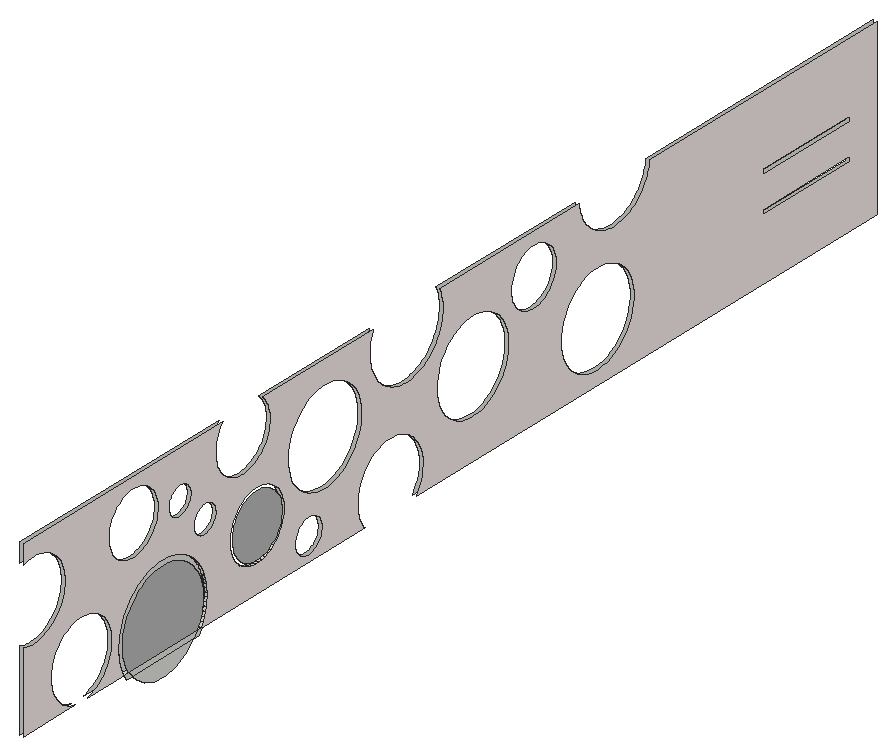
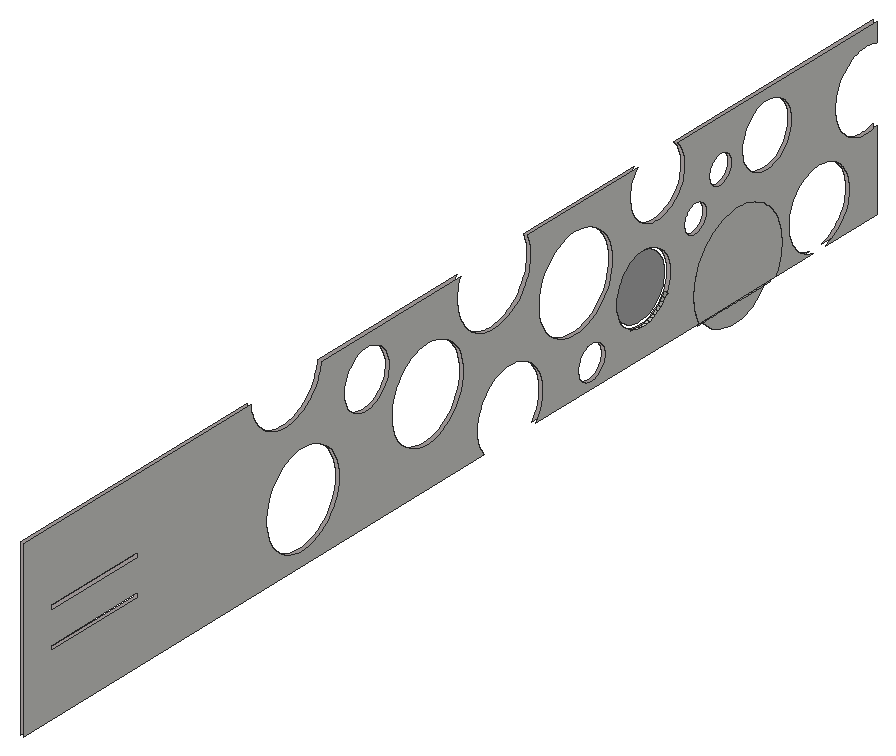
# SketchUp Ruby script. Lengths in inches.
U = 1.inch
M = Sketchup.active_model
def pt(a) = Geom::Point3d.new(a.map { |v| v * U })
def face(e, loops, mat)
  f = e.add_face(loops[0].map { |a| pt(a) })
  loops[1..].each { |l| e.add_face(l.map { |a| pt(a) }).erase! }
  f.material = f.back_material = mat if mat
  f
end
# faces: each face lists its corners as indices into pts; further lists are holes
def faces(e, pts, list, mat = nil) = list.each { |f| face(e, (f[0].is_a?(Array) ? f : [f]).map { |l| l.map { |i| pts[i] } }, mat) }
# xy, xz, yz: faces in a plane at the given z, y or x. An outline is a flat list of corners, or four numbers for a rectangle; further outlines are holes
def ring(l) = l.size == 4 ? [[l[0], l[1]], [l[2], l[1]], [l[2], l[3]], [l[0], l[3]]] : l.each_slice(2).to_a
def flat(e, list, mat, &to3) = list.each { |f| face(e, (f[0].is_a?(Array) ? f : [f]).map { |l| ring(l).map { |u, v| to3.(u, v) } }, mat) }
def xy(e, z, list, mat = nil) = flat(e, list, mat) { |x, y| [x, y, z] }
def xz(e, y, list, mat = nil) = flat(e, list, mat) { |x, z| [x, y, z] }
def yz(e, x, list, mat = nil) = flat(e, list, mat) { |y, z| [x, y, z] }
def lines(e, pts, list) = list.each { |a, b| e.add_line(pt(pts[a]), pt(pts[b])) }
# prism: a flat outline (further loops are holes) pulled along v
def prism(e, loops, v, mat = nil)
  f = face(e, loops, mat); d = Geom::Vector3d.new(v.map { |x| x * U })
  f.pushpull(f.normal.samedirection?(d) ? d.length : -d.length)
end
def box(e, o, s, mat = nil) = prism(e, [[o, [o[0] + s[0], o[1], o[2]], [o[0] + s[0], o[1] + s[1], o[2]], [o[0], o[1] + s[1], o[2]]]], [0, 0, s[2]], mat)
def at(x, y, z, deg = 0) = Geom::Transformation.translation(pt([x, y, z])) * Geom::Transformation.rotation(ORIGIN, Z_AXIS, deg.degrees)
def axes(o, x, y, z) = Geom::Transformation.new([*x, 0, *y, 0, *z, 0, *pt(o).to_a, 1])
def part(name) = M.definitions.add(name)
# library, detail: a bought-in or finely detailed component or shape, given as its bounding box
def library(name, o, s) = part(name).tap { |d| box(d.entities, o, s) }
def detail(e, o, s) = box(e.add_group.entities, o, s)
def put(e, d, t, mat = nil) = e.add_instance(d, t).tap { |i| i.material = mat if mat }
def group(e, t, mat = nil) = e.add_group.tap { |g| g.transformation = t; g.material = mat if mat }.entities
root = M.entities
M.materials.add("Generic\#2").color = [246, 234, 234]
M.materials.add("[Mirror 01]").color = [185, 185, 185]
xy(root,46.5,[[9,53.23,10.6875,94.93]])
yz(root,9,[[[0.4375,46.5,0.4375,80.35,1.09,80.07,2.53,79.73,3.92,79.53,5.3125,79.45,6.71,79.48,8.1,79.625,9.48,79.89,10.83,80.27,12.14,80.75,13.4,81.35,14.61,82.05,15.76,82.85,16.84,83.74,17.84,84.72,18.75,85.78,19.58,86.91,20.3,88.11,20.92,89.36,21.44,90.66,21.84,92,22.14,93.37,22.3125,94.76,22.375,96.15,22.32,97.55,22.14,98.94,21.85,100.31,21.45,101.65,20.9375,102.95,20.32,104.21,19.6,105.4,18.78,106.54,17.86,107.6,16.87,108.58,15.79,109.47,14.64,110.28,13.43,110.98,12.17,111.58,10.86,112.07,9.51,112.45,8.14,112.71,6.75,112.87,5.35,112.9,3.95,112.82,2.57,112.62,1.18,112.3,0.4375,112.04,0.4375,120,106.01,120,105.5,119.44,104.63,118.3125,103.89,117.11,103.26,115.84,102.75,114.51,102.38,113.14,102.14,111.74,102.04,110.32,102.07,108.91,102.24,107.5,102.55,106.11,102.99,104.76,103.56,103.46,104.25,102.22,105.05,101.05,105.97,99.97,106.98,98.97,108.09,98.09,109.28,97.31,110.53,96.65,111.85,96.11,113.21,95.71,114.6,95.43,116.01,95.3,117.43,95.3,118.85,95.43,120.24,95.71,121.6,96.11,122.91,96.65,124.17,97.31,125.36,98.09,126.46,98.97,127.48,99.97,128.4,101.05,129.2,102.22,129.89,103.46,130.46,104.76,130.9,106.11,131.2,107.5,131.375,108.91,131.41,110.32,131.31,111.74,131.07,113.14,130.69,114.51,130.19,115.84,129.5625,117.11,128.8125,118.3125,127.95,119.44,127.43,120,185.75,120,185.61,119.71,185.04,118.26,184.59,116.77,184.25,115.24,184.04,113.7,183.95,112.14,183.99,110.58,184.15,109.02,184.43,107.49,184.84,105.98,185.36,104.51,185.99,103.08,186.74,101.71,187.6,100.41,188.55,99.17,189.6,98.02,190.74,96.95,191.96,95.97,193.25,95.1,194.61,94.33,196.02,93.67,197.48,93.12,198.99,92.69,200.52,92.38,202.07,92.2,203.625,92.14,205.19,92.2,206.74,92.38,208.27,92.69,209.77,93.12,211.23,93.67,212.64,94.33,214,95.1,215.29,95.97,216.51,96.95,217.65,98.02,218.7,99.17,219.66,100.41,220.51,101.71,221.26,103.08,221.89,104.51,222.42,105.98,222.82,107.49,223.1,109.02,223.26,110.58,223.3,112.14,223.21,113.7,223,115.24,222.66,116.77,222.21,118.26,221.64,119.71,221.5,120,295.22,120,295.4375,118.67,295.65,117.68,295.91,116.7,296.23,115.73,296.6,114.78,297.02,113.85,297.49,112.95,298,112.07,298.56,111.23,299.17,110.41,299.82,109.625,300.51,108.875,301.24,108.17,302,107.5,302.8,106.87,303.63,106.28,304.49,105.74,305.38,105.25,306.3,104.8,307.24,104.41,308.19,104.06,309.17,103.77,310.15,103.52,311.15,103.34,312.16,103.2,313.18,103.12,314.19,103.09,315.21,103.12,316.22,103.2,317.23,103.34,318.23,103.52,319.22,103.77,320.19,104.06,321.15,104.41,322.09,104.8,323,105.25,323.89,105.74,324.75,106.28,325.59,106.87,326.39,107.5,327.15,108.17,327.88,108.875,328.57,109.625,329.22,110.41,329.82,111.23,330.38,112.07,330.9,112.95,331.37,113.85,331.79,114.78,332.15,115.73,332.47,116.7,332.74,117.68,332.95,118.67,333.16,120,453.375,120,453.375,46.5,209.04,46.5,209.84,47.59,210.84,49.33,211.63,51.17,212.21,53.09,212.56,55.07,212.6875,57.07,212.58,59.07,212.25,61.05,211.7,62.97,210.93,64.82,209.95,66.58,208.78,68.2,207.4375,69.69,205.93,71.01,204.28,72.15,202.51,73.1,200.65,73.84,198.71,74.36,196.73,74.65,194.73,74.72,192.73,74.5625,190.76,74.18,188.85,73.57,187.02,72.74,185.3,71.72,183.7,70.5,182.26,69.11,180.98,67.57,179.89,65.89,178.99,64.1,178.31,62.21,177.84,60.26,177.6,58.27,177.59,56.27,177.81,54.27,178.25,52.32,178.91,50.42,179.79,48.62,180.86,46.93,181.21,46.5,94.93,46.5,94.96,46.54,95.8,48.26,96.46,49.91,96.99,51.61,97.4,53.35,97.67,55.1,97.8125,56.88,97.82,58.66,97.7,60.4375,97.44,62.2,97.05,63.93,96.53,65.64,95.89,67.3,95.125,68.91,94.24,70.45,93.24,71.92,92.14,73.32,90.93,74.63,89.63,75.84,88.24,76.96,86.77,77.97,85.23,78.86,83.63,79.64,81.97,80.29,80.27,80.82,78.54,81.22,76.78,81.49,75,81.625,73.22,81.63,71.45,81.5,69.69,81.23,67.95,80.84,66.25,80.32,64.59,79.67,62.98,78.9,61.44,78.01,59.97,77,58.58,75.89,57.27,74.68,56.0625,73.38,54.95,71.99,53.95,70.52,53.06,68.97,52.29,67.37,51.64,65.71,51.12,64.01,50.72,62.27,50.46,60.51,50.33,58.74,50.33,56.96,50.47,55.18,50.73,53.42,51.13,51.69,51.66,49.99,52.32,48.33,53.12,46.68,53.23,46.5,34.125,46.5,35.01,46.69,36.33,47.11,37.61,47.625,38.84,48.25,40.02,48.99,41.125,49.8125,42.16,50.73,43.11,51.73,43.98,52.8125,44.75,53.96,45.42,55.17,45.98,56.4375,46.43,57.74,46.78,59.08,47,60.45,47.12,61.83,47.11,63.21,46.99,64.59,46.75,65.95,46.39,67.29,45.93,68.59,45.35,69.85,44.67,71.05,43.89,72.19,43.02,73.27,42.06,74.26,41.01,75.17,39.9,75.99,38.72,76.71,37.48,77.32,36.19,77.83,34.87,78.23,33.51,78.52,32.14,78.6875,30.76,78.74,29.38,78.68,28.01,78.49,26.66,78.2,25.34,77.79,24.05,77.26,22.82,76.64,21.65,75.91,20.54,75.08,19.5,74.16,18.55,73.16,17.6875,72.08,16.92,70.93,16.25,69.72,15.68,68.45,15.23,67.15,14.89,65.81,14.66,64.44,14.55,63.06,14.55,61.68,14.68,60.3,14.92,58.94,15.27,57.6,15.74,56.3,16.3125,55.04,16.99,53.84,17.77,52.7,18.65,51.625,19.61,50.63,20.65,49.72,21.77,48.9,22.95,48.18,24.1875,47.57,25.47,47.06,26.8,46.66,27.54,46.5],[160.49,70.77,162.75,70.92,164.98,71.34,167.15,72,169.22,72.9,171.18,74.04,173,75.39,174.65,76.95,176.12,78.68,177.38,80.56,178.41,82.58,179.21,84.7,179.76,86.9,180.06,89.14,180.1,91.41,179.88,93.66,179.4,95.88,178.68,98.03,177.71,100.08,176.52,102.01,175.12,103.78,173.52,105.39,171.75,106.81,169.83,108.01,167.78,108.99,165.64,109.72,163.43,110.21,161.17,110.44,158.91,110.42,156.66,110.14,154.46,109.6,152.33,108.8125,150.31,107.79,148.42,106.54,146.68,105.09,145.12,103.44,143.75,101.63,142.61,99.68,141.6875,97.61,141.01,95.44,140.59,93.22,140.42,90.96,140.51,88.69,140.86,86.45,141.46,84.27,142.3,82.17,143.38,80.17,144.68,78.32,146.1875,76.62,147.875,75.11,149.72,73.8,151.71,72.71,153.81,71.85,155.99,71.23,158.23,70.87],[305.99,52.23,308.22,52.44,310.42,52.9,312.54,53.61,314.58,54.5625,316.49,55.74,318.25,57.12,319.85,58.7,321.26,60.44,322.45,62.34,323.43,64.36,324.17,66.48,324.66,68.67,324.89,70.9,324.875,73.14,324.6,75.37,324.08,77.55,323.31,79.66,322.3,81.66,321.07,83.54,319.64,85.27,318.02,86.82,316.23,88.17,314.3,89.31,312.25,90.23,310.11,90.91,307.91,91.33,305.68,91.51,303.43,91.43,301.22,91.09,299.05,90.5,296.97,89.67,294.99,88.61,293.15,87.33,291.47,85.85,289.96,84.18,288.66,82.36,287.57,80.39,286.71,78.32,286.1,76.16,285.73,73.95,285.625,71.71,285.77,69.47,286.17,67.26,286.82,65.12,287.71,63.06,288.83,61.11,290.16,59.31,291.69,57.67,293.4,56.21,295.26,54.96,297.25,53.93,299.35,53.13,301.52,52.58,303.74,52.28],[239.61,63.57,241.81,63.77,243.97,64.23,246.06,64.93,248.0625,65.86,249.94,67.02,251.68,68.38,253.25,69.93,254.64,71.65,255.82,73.52,256.77,75.51,257.5,77.59,257.98,79.75,258.22,81.94,258.2,84.15,257.93,86.34,257.41,88.49,256.66,90.5625,255.67,92.54,254.46,94.39,253.05,96.08,251.45,97.61,249.69,98.95,247.79,100.07,245.78,100.97,243.67,101.64,241.5,102.06,239.3,102.23,237.09,102.15,234.91,101.82,232.78,101.24,230.73,100.42,228.78,99.38,226.97,98.12,225.3125,96.66,223.83,95.02,222.55,93.22,221.48,91.29,220.64,89.25,220.03,87.125,219.67,84.95,219.5625,82.74,219.71,80.54,220.1,78.37,220.74,76.25,221.61,74.22,222.71,72.3125,224.03,70.53,225.53,68.92,227.21,67.49,229.05,66.25,231.01,65.24,233.07,64.45,235.21,63.91,237.4,63.61],[123.83,58.04,125.5,58.09,127.15,58.33,128.76,58.76,130.32,59.36,131.8,60.15,133.17,61.09,134.4375,62.1875,135.5625,63.42,136.54,64.77,137.36,66.23,138.01,67.77,138.48,69.375,138.76,71.02,138.85,72.69,138.75,74.36,138.47,76,137.99,77.61,137.34,79.14,136.52,80.6,135.53,81.95,134.4,83.18,133.14,84.27,131.75,85.21,130.28,85.99,128.72,86.59,127.1,87.01,125.45,87.25,123.78,87.29,122.11,87.15,120.48,86.8125,118.89,86.29,117.37,85.6,115.94,84.73,114.62,83.71,113.42,82.54,112.37,81.25,111.47,79.84,110.73,78.34,110.17,76.76,109.8,75.14,109.61,73.48,109.61,71.81,109.8,70.15,110.1875,68.52,110.75,66.95,111.49,65.45,112.4,64.04,113.46,62.75,114.66,61.59,115.98,60.57,117.41,59.71,118.93,59.02,120.52,58.51,122.16,58.18],[59.06,89.02,60.53,89.17,61.96,89.47,63.36,89.93,64.7,90.54,65.96,91.29,67.13,92.18,68.2,93.1875,69.15,94.31,69.97,95.53,70.65,96.83,71.18,98.2,71.5625,99.62,71.78,101.07,71.84,102.54,71.74,104,71.48,105.45,71.06,106.86,70.49,108.21,69.77,109.49,68.92,110.6875,67.93,111.78,66.84,112.76,65.64,113.62,64.36,114.33,63.01,114.9,61.6,115.32,60.15,115.58,58.6875,115.68,57.22,115.62,55.77,115.4,54.35,115.02,52.98,114.48,51.68,113.8,50.46,112.98,49.34,112.03,48.33,110.96,47.44,109.79,46.69,108.53,46.08,107.19,45.625,105.8,45.32,104.36,45.18,102.89,45.2,101.43,45.39,99.97,45.73,98.54,46.22,97.16,46.87,95.84,47.66,94.6,48.58,93.45,49.62,92.41,50.76,91.49,52,90.71,53.32,90.0625,54.71,89.57,56.14,89.23,57.6,89.04],[271.5625,90.52,272.95,90.625,274.32,90.89,275.64,91.3,276.91,91.86,278.11,92.57,279.22,93.41,280.23,94.37,281.125,95.43,281.89,96.59,282.52,97.84,283,99.14,283.33,100.49,283.5,101.87,283.52,103.26,283.37,104.65,283.07,106,282.62,107.32,282.02,108.57,281.28,109.75,280.41,110.84,279.42,111.82,278.33,112.68,277.15,113.41,275.89,114,274.57,114.45,273.21,114.74,271.83,114.87,270.4375,114.85,269.06,114.66,267.71,114.32,266.41,113.83,265.17,113.2,264.01,112.43,262.95,111.53,262,110.51,261.17,109.4,260.47,108.19,259.92,106.92,259.51,105.59,259.26,104.22,259.17,102.83,259.23,101.44,259.45,100.07,259.83,98.73,260.36,97.44,261.03,96.23,261.83,95.09,262.76,94.06,263.8,93.13,264.94,92.34,266.17,91.67,267.46,91.16,268.8,90.79,270.17,90.58],[152.02,49.25,152.83,49.33,153.61,49.5,154.38,49.76,155.11,50.09,155.8,50.51,156.44,51,157.02,51.55,157.54,52.17,157.99,52.84,158.36,53.56,158.65,54.31,158.85,55.09,158.97,55.88,159,56.6875,158.94,57.49,158.79,58.28,158.56,59.06,158.24,59.8,157.85,60.5,157.375,61.15,156.84,61.75,156.23,62.28,155.58,62.75,154.87,63.14,154.13,63.45,153.35,63.67,152.5625,63.81,151.76,63.87,150.95,63.83,150.16,63.7,149.38,63.49,148.63,63.2,147.92,62.82,147.25,62.37,146.64,61.84,146.09,61.26,145.61,60.61,145.2,59.92,144.87,59.18,144.62,58.42,144.46,57.625,144.38,56.82,144.4,56.02,144.5,55.22,144.69,54.4375,144.97,53.68,145.32,52.96,145.76,52.28,146.26,51.65,146.84,51.09,147.47,50.59,148.15,50.16,148.875,49.81,149.63,49.54,150.42,49.36,151.22,49.26],[83.09,93.93,83.68,93.94,84.26,94.02,84.84,94.15,85.4,94.33,85.9375,94.57,86.45,94.86,86.93,95.2,87.38,95.58,87.79,96.01,88.16,96.47,88.48,96.97,88.75,97.49,88.97,98.04,89.14,98.6,89.25,99.18,89.3,99.77,89.3,100.36,89.24,100.95,89.12,101.53,88.95,102.09,88.72,102.64,88.44,103.16,88.12,103.65,87.75,104.11,87.33,104.53,86.88,104.9,86.39,105.24,85.875,105.52,85.33,105.75,84.77,105.93,84.19,106.06,83.61,106.125,83.02,106.13,82.43,106.09,81.85,105.99,81.28,105.83,80.73,105.62,80.2,105.35,79.7,105.04,79.24,104.68,78.81,104.27,78.42,103.83,78.07,103.35,77.78,102.84,77.53,102.3,77.34,101.74,77.2,101.17,77.12,100.59,77.09,100,77.125,99.41,77.21,98.82,77.36,98.25,77.56,97.7,77.81,97.16,78.11,96.66,78.46,96.18,78.85,95.74,79.29,95.34,79.76,94.99,80.26,94.68,80.79,94.42,81.34,94.21,81.91,94.0625,82.5,93.97],[96.4375,81.13,97.02,81.15,97.6,81.23,98.17,81.35,98.72,81.54,99.26,81.77,99.76,82.06,100.24,82.39,100.68,82.77,101.09,83.19,101.45,83.65,101.77,84.14,102.04,84.66,102.25,85.2,102.42,85.76,102.53,86.33,102.58,86.91,102.58,87.49,102.52,88.07,102.4,88.64,102.23,89.2,102.01,89.74,101.73,90.26,101.41,90.74,101.04,91.19,100.64,91.61,100.1875,91.98,99.71,92.3125,99.19,92.59,98.66,92.82,98.1,93,97.53,93.12,96.95,93.1875,96.37,93.2,95.79,93.15,95.22,93.05,94.65,92.9,94.11,92.6875,93.59,92.42,93.1,92.11,92.63,91.76,92.21,91.36,91.83,90.92,91.49,90.45,91.19,89.94,90.95,89.41,90.76,88.86,90.625,88.29,90.54,87.72,90.52,87.13,90.55,86.55,90.64,85.98,90.78,85.41,90.98,84.86,91.22,84.33,91.52,83.83,91.87,83.36,92.26,82.93,92.6875,82.53,93.15,82.18,93.65,81.88,94.17,81.62,94.72,81.42,95.28,81.27,95.86,81.17],[393.02,72.8125,439.14,75],[393.02,88.25,439.14,90.4375]],[53.23,46.5,94.93,46.5,94.96,46.54,95.8,48.26,96.46,49.91,96.99,51.61,97.4,53.35,97.67,55.1,97.8125,56.88,97.82,58.66,97.7,60.4375,97.44,62.2,97.05,63.93,96.53,65.64,95.89,67.3,95.125,68.91,94.24,70.45,93.24,71.92,92.14,73.32,90.93,74.63,89.63,75.84,88.24,76.96,86.77,77.97,85.23,78.86,83.63,79.64,81.97,80.29,80.27,80.82,78.54,81.22,76.78,81.49,75,81.625,73.22,81.63,71.45,81.5,69.69,81.23,67.95,80.84,66.25,80.32,64.59,79.67,62.98,78.9,61.44,78.01,59.97,77,58.58,75.89,57.27,74.68,56.0625,73.38,54.95,71.99,53.95,70.52,53.06,68.97,52.29,67.37,51.64,65.71,51.12,64.01,50.72,62.27,50.46,60.51,50.33,58.74,50.33,56.96,50.47,55.18,50.73,53.42,51.13,51.69,51.66,49.99,52.32,48.33,53.12,46.68]])
yz(root,10.6875,[[75.53,36.56,81,37.66,86,40.14,90.18,43.83,90.37,44.12,57.96,44.12,60.03,41.77,64.67,38.68,69.96,36.9],[54.76,44.12,57.96,44.12,56.33,45.96,56.0625,46.5,53.23,46.5],[57.96,44.12,90.37,44.12,91.96,46.5,56.0625,46.5,56.33,45.96],[90.37,44.12,93.15,44.12,94.93,46.5,91.96,46.5]])
yz(root,10.6875,[[[0.4375,46.5,27.54,46.5,26.8,46.66,25.47,47.06,24.1875,47.57,22.95,48.18,21.77,48.9,20.65,49.72,19.61,50.63,18.65,51.625,17.77,52.7,16.99,53.84,16.3125,55.04,15.74,56.3,15.27,57.6,14.92,58.94,14.68,60.3,14.55,61.68,14.55,63.06,14.66,64.44,14.89,65.81,15.23,67.15,15.68,68.45,16.25,69.72,16.92,70.93,17.6875,72.08,18.55,73.16,19.5,74.16,20.54,75.08,21.65,75.91,22.82,76.64,24.05,77.26,25.34,77.79,26.66,78.2,28.01,78.49,29.38,78.68,30.76,78.74,32.14,78.6875,33.51,78.52,34.87,78.23,36.19,77.83,37.48,77.32,38.72,76.71,39.9,75.99,41.01,75.17,42.06,74.26,43.02,73.27,43.89,72.19,44.67,71.05,45.35,69.85,45.93,68.59,46.39,67.29,46.75,65.95,46.99,64.59,47.11,63.21,47.12,61.83,47,60.45,46.78,59.08,46.43,57.74,45.98,56.4375,45.42,55.17,44.75,53.96,43.98,52.8125,43.11,51.73,42.16,50.73,41.125,49.8125,40.02,48.99,38.84,48.25,37.61,47.625,36.33,47.11,35.01,46.69,34.125,46.5,53.23,46.5,53.12,46.68,52.32,48.33,51.66,49.99,51.13,51.69,50.73,53.42,50.47,55.18,50.33,56.96,50.33,58.74,50.46,60.51,50.72,62.27,51.12,64.01,51.64,65.71,52.29,67.37,53.06,68.97,53.95,70.52,54.95,71.99,56.0625,73.38,57.27,74.68,58.58,75.89,59.97,77,61.44,78.01,62.98,78.9,64.59,79.67,66.25,80.32,67.95,80.84,69.69,81.23,71.45,81.5,73.22,81.63,75,81.625,76.78,81.49,78.54,81.22,80.27,80.82,81.97,80.29,83.63,79.64,85.23,78.86,86.77,77.97,88.24,76.96,89.63,75.84,90.93,74.63,92.14,73.32,93.24,71.92,94.24,70.45,95.125,68.91,95.89,67.3,96.53,65.64,97.05,63.93,97.44,62.2,97.7,60.4375,97.82,58.66,97.8125,56.88,97.67,55.1,97.4,53.35,96.99,51.61,96.46,49.91,95.8,48.26,94.96,46.54,94.93,46.5,181.21,46.5,180.86,46.93,179.79,48.62,178.91,50.42,178.25,52.32,177.81,54.27,177.59,56.27,177.6,58.27,177.84,60.26,178.31,62.21,178.99,64.1,179.89,65.89,180.98,67.57,182.26,69.11,183.7,70.5,185.3,71.72,187.02,72.74,188.85,73.57,190.76,74.18,192.73,74.5625,194.73,74.72,196.73,74.65,198.71,74.36,200.65,73.84,202.51,73.1,204.28,72.15,205.93,71.01,207.4375,69.69,208.78,68.2,209.95,66.58,210.93,64.82,211.7,62.97,212.25,61.05,212.58,59.07,212.6875,57.07,212.56,55.07,212.21,53.09,211.63,51.17,210.84,49.33,209.84,47.59,209.04,46.5,453.375,46.5,453.375,120,333.16,120,332.95,118.67,332.74,117.68,332.47,116.7,332.15,115.73,331.79,114.78,331.37,113.85,330.9,112.95,330.38,112.07,329.82,111.23,329.22,110.41,328.57,109.625,327.88,108.875,327.15,108.17,326.39,107.5,325.59,106.87,324.75,106.28,323.89,105.74,323,105.25,322.09,104.8,321.15,104.41,320.19,104.06,319.22,103.77,318.23,103.52,317.23,103.34,316.22,103.2,315.21,103.12,314.19,103.09,313.18,103.12,312.16,103.2,311.15,103.34,310.15,103.52,309.17,103.77,308.19,104.06,307.24,104.41,306.3,104.8,305.38,105.25,304.49,105.74,303.63,106.28,302.8,106.87,302,107.5,301.24,108.17,300.51,108.875,299.82,109.625,299.17,110.41,298.56,111.23,298,112.07,297.49,112.95,297.02,113.85,296.6,114.78,296.23,115.73,295.91,116.7,295.65,117.68,295.4375,118.67,295.22,120,221.5,120,221.64,119.71,222.21,118.26,222.66,116.77,223,115.24,223.21,113.7,223.3,112.14,223.26,110.58,223.1,109.02,222.82,107.49,222.42,105.98,221.89,104.51,221.26,103.08,220.51,101.71,219.66,100.41,218.7,99.17,217.65,98.02,216.51,96.95,215.29,95.97,214,95.1,212.64,94.33,211.23,93.67,209.77,93.12,208.27,92.69,206.74,92.38,205.19,92.2,203.625,92.14,202.07,92.2,200.52,92.38,198.99,92.69,197.48,93.12,196.02,93.67,194.61,94.33,193.25,95.1,191.96,95.97,190.74,96.95,189.6,98.02,188.55,99.17,187.6,100.41,186.74,101.71,185.99,103.08,185.36,104.51,184.84,105.98,184.43,107.49,184.15,109.02,183.99,110.58,183.95,112.14,184.04,113.7,184.25,115.24,184.59,116.77,185.04,118.26,185.61,119.71,185.75,120,127.43,120,127.95,119.44,128.8125,118.3125,129.5625,117.11,130.19,115.84,130.69,114.51,131.07,113.14,131.31,111.74,131.41,110.32,131.375,108.91,131.2,107.5,130.9,106.11,130.46,104.76,129.89,103.46,129.2,102.22,128.4,101.05,127.48,99.97,126.46,98.97,125.36,98.09,124.17,97.31,122.91,96.65,121.6,96.11,120.24,95.71,118.85,95.43,117.43,95.3,116.01,95.3,114.6,95.43,113.21,95.71,111.85,96.11,110.53,96.65,109.28,97.31,108.09,98.09,106.98,98.97,105.97,99.97,105.05,101.05,104.25,102.22,103.56,103.46,102.99,104.76,102.55,106.11,102.24,107.5,102.07,108.91,102.04,110.32,102.14,111.74,102.38,113.14,102.75,114.51,103.26,115.84,103.89,117.11,104.63,118.3125,105.5,119.44,106.01,120,0.4375,120,0.4375,112.04,1.18,112.3,2.57,112.62,3.95,112.82,5.35,112.9,6.75,112.87,8.14,112.71,9.51,112.45,10.86,112.07,12.17,111.58,13.43,110.98,14.64,110.28,15.79,109.47,16.87,108.58,17.86,107.6,18.78,106.54,19.6,105.4,20.32,104.21,20.9375,102.95,21.45,101.65,21.85,100.31,22.14,98.94,22.32,97.55,22.375,96.15,22.3125,94.76,22.14,93.37,21.84,92,21.44,90.66,20.92,89.36,20.3,88.11,19.58,86.91,18.75,85.78,17.84,84.72,16.84,83.74,15.76,82.85,14.61,82.05,13.4,81.35,12.14,80.75,10.83,80.27,9.48,79.89,8.1,79.625,6.71,79.48,5.3125,79.45,3.92,79.53,2.53,79.73,1.09,80.07,0.4375,80.35],[160.49,70.77,158.23,70.87,155.99,71.23,153.81,71.85,151.71,72.71,149.72,73.8,147.875,75.11,146.1875,76.62,144.68,78.32,143.38,80.17,142.3,82.17,141.46,84.27,140.86,86.45,140.51,88.69,140.42,90.96,140.59,93.22,141.01,95.44,141.6875,97.61,142.61,99.68,143.75,101.63,145.12,103.44,146.68,105.09,148.42,106.54,150.31,107.79,152.33,108.8125,154.46,109.6,156.66,110.14,158.91,110.42,161.17,110.44,163.43,110.21,165.64,109.72,167.78,108.99,169.83,108.01,171.75,106.81,173.52,105.39,175.12,103.78,176.52,102.01,177.71,100.08,178.68,98.03,179.4,95.88,179.88,93.66,180.1,91.41,180.06,89.14,179.76,86.9,179.21,84.7,178.41,82.58,177.38,80.56,176.12,78.68,174.65,76.95,173,75.39,171.18,74.04,169.22,72.9,167.15,72,164.98,71.34,162.75,70.92],[305.99,52.23,303.74,52.28,301.52,52.58,299.35,53.13,297.25,53.93,295.26,54.96,293.4,56.21,291.69,57.67,290.16,59.31,288.83,61.11,287.71,63.06,286.82,65.12,286.17,67.26,285.77,69.47,285.625,71.71,285.73,73.95,286.1,76.16,286.71,78.32,287.57,80.39,288.66,82.36,289.96,84.18,291.47,85.85,293.15,87.33,294.99,88.61,296.97,89.67,299.05,90.5,301.22,91.09,303.43,91.43,305.68,91.51,307.91,91.33,310.11,90.91,312.25,90.23,314.3,89.31,316.23,88.17,318.02,86.82,319.64,85.27,321.07,83.54,322.3,81.66,323.31,79.66,324.08,77.55,324.6,75.37,324.875,73.14,324.89,70.9,324.66,68.67,324.17,66.48,323.43,64.36,322.45,62.34,321.26,60.44,319.85,58.7,318.25,57.12,316.49,55.74,314.58,54.5625,312.54,53.61,310.42,52.9,308.22,52.44],[239.61,63.57,237.4,63.61,235.21,63.91,233.07,64.45,231.01,65.24,229.05,66.25,227.21,67.49,225.53,68.92,224.03,70.53,222.71,72.3125,221.61,74.22,220.74,76.25,220.1,78.37,219.71,80.54,219.5625,82.74,219.67,84.95,220.03,87.125,220.64,89.25,221.48,91.29,222.55,93.22,223.83,95.02,225.3125,96.66,226.97,98.12,228.78,99.38,230.73,100.42,232.78,101.24,234.91,101.82,237.09,102.15,239.3,102.23,241.5,102.06,243.67,101.64,245.78,100.97,247.79,100.07,249.69,98.95,251.45,97.61,253.05,96.08,254.46,94.39,255.67,92.54,256.66,90.5625,257.41,88.49,257.93,86.34,258.2,84.15,258.22,81.94,257.98,79.75,257.5,77.59,256.77,75.51,255.82,73.52,254.64,71.65,253.25,69.93,251.68,68.38,249.94,67.02,248.0625,65.86,246.06,64.93,243.97,64.23,241.81,63.77],[123.83,58.04,122.16,58.18,120.52,58.51,118.93,59.02,117.41,59.71,115.98,60.57,114.66,61.59,113.46,62.75,112.4,64.04,111.49,65.45,110.75,66.95,110.1875,68.52,109.8,70.15,109.61,71.81,109.61,73.48,109.8,75.14,110.17,76.76,110.73,78.34,111.47,79.84,112.37,81.25,113.42,82.54,114.62,83.71,115.94,84.73,117.37,85.6,118.89,86.29,120.48,86.8125,122.11,87.15,123.78,87.29,125.45,87.25,127.1,87.01,128.72,86.59,130.28,85.99,131.75,85.21,133.14,84.27,134.4,83.18,135.53,81.95,136.52,80.6,137.34,79.14,137.99,77.61,138.47,76,138.75,74.36,138.85,72.69,138.76,71.02,138.48,69.375,138.01,67.77,137.36,66.23,136.54,64.77,135.5625,63.42,134.4375,62.1875,133.17,61.09,131.8,60.15,130.32,59.36,128.76,58.76,127.15,58.33,125.5,58.09],[59.06,89.02,57.6,89.04,56.14,89.23,54.71,89.57,53.32,90.0625,52,90.71,50.76,91.49,49.62,92.41,48.58,93.45,47.66,94.6,46.87,95.84,46.22,97.16,45.73,98.54,45.39,99.97,45.2,101.43,45.18,102.89,45.32,104.36,45.625,105.8,46.08,107.19,46.69,108.53,47.44,109.79,48.33,110.96,49.34,112.03,50.46,112.98,51.68,113.8,52.98,114.48,54.35,115.02,55.77,115.4,57.22,115.62,58.6875,115.68,60.15,115.58,61.6,115.32,63.01,114.9,64.36,114.33,65.64,113.62,66.84,112.76,67.93,111.78,68.92,110.6875,69.77,109.49,70.49,108.21,71.06,106.86,71.48,105.45,71.74,104,71.84,102.54,71.78,101.07,71.5625,99.62,71.18,98.2,70.65,96.83,69.97,95.53,69.15,94.31,68.2,93.1875,67.13,92.18,65.96,91.29,64.7,90.54,63.36,89.93,61.96,89.47,60.53,89.17],[271.5625,90.52,270.17,90.58,268.8,90.79,267.46,91.16,266.17,91.67,264.94,92.34,263.8,93.13,262.76,94.06,261.83,95.09,261.03,96.23,260.36,97.44,259.83,98.73,259.45,100.07,259.23,101.44,259.17,102.83,259.26,104.22,259.51,105.59,259.92,106.92,260.47,108.19,261.17,109.4,262,110.51,262.95,111.53,264.01,112.43,265.17,113.2,266.41,113.83,267.71,114.32,269.06,114.66,270.4375,114.85,271.83,114.87,273.21,114.74,274.57,114.45,275.89,114,277.15,113.41,278.33,112.68,279.42,111.82,280.41,110.84,281.28,109.75,282.02,108.57,282.62,107.32,283.07,106,283.37,104.65,283.52,103.26,283.5,101.87,283.33,100.49,283,99.14,282.52,97.84,281.89,96.59,281.125,95.43,280.23,94.37,279.22,93.41,278.11,92.57,276.91,91.86,275.64,91.3,274.32,90.89,272.95,90.625],[152.02,49.25,151.22,49.26,150.42,49.36,149.63,49.54,148.875,49.81,148.15,50.16,147.47,50.59,146.84,51.09,146.26,51.65,145.76,52.28,145.32,52.96,144.97,53.68,144.69,54.4375,144.5,55.22,144.4,56.02,144.38,56.82,144.46,57.625,144.62,58.42,144.87,59.18,145.2,59.92,145.61,60.61,146.09,61.26,146.64,61.84,147.25,62.37,147.92,62.82,148.63,63.2,149.38,63.49,150.16,63.7,150.95,63.83,151.76,63.87,152.5625,63.81,153.35,63.67,154.13,63.45,154.87,63.14,155.58,62.75,156.23,62.28,156.84,61.75,157.375,61.15,157.85,60.5,158.24,59.8,158.56,59.06,158.79,58.28,158.94,57.49,159,56.6875,158.97,55.88,158.85,55.09,158.65,54.31,158.36,53.56,157.99,52.84,157.54,52.17,157.02,51.55,156.44,51,155.8,50.51,155.11,50.09,154.38,49.76,153.61,49.5,152.83,49.33],[83.09,93.93,82.5,93.97,81.91,94.0625,81.34,94.21,80.79,94.42,80.26,94.68,79.76,94.99,79.29,95.34,78.85,95.74,78.46,96.18,78.11,96.66,77.81,97.16,77.56,97.7,77.36,98.25,77.21,98.82,77.125,99.41,77.09,100,77.12,100.59,77.2,101.17,77.34,101.74,77.53,102.3,77.78,102.84,78.07,103.35,78.42,103.83,78.81,104.27,79.24,104.68,79.7,105.04,80.2,105.35,80.73,105.62,81.28,105.83,81.85,105.99,82.43,106.09,83.02,106.13,83.61,106.125,84.19,106.06,84.77,105.93,85.33,105.75,85.875,105.52,86.39,105.24,86.88,104.9,87.33,104.53,87.75,104.11,88.12,103.65,88.44,103.16,88.72,102.64,88.95,102.09,89.12,101.53,89.24,100.95,89.3,100.36,89.3,99.77,89.25,99.18,89.14,98.6,88.97,98.04,88.75,97.49,88.48,96.97,88.16,96.47,87.79,96.01,87.38,95.58,86.93,95.2,86.45,94.86,85.9375,94.57,85.4,94.33,84.84,94.15,84.26,94.02,83.68,93.94],[96.4375,81.13,95.86,81.17,95.28,81.27,94.72,81.42,94.17,81.62,93.65,81.88,93.15,82.18,92.6875,82.53,92.26,82.93,91.87,83.36,91.52,83.83,91.22,84.33,90.98,84.86,90.78,85.41,90.64,85.98,90.55,86.55,90.52,87.13,90.54,87.72,90.625,88.29,90.76,88.86,90.95,89.41,91.19,89.94,91.49,90.45,91.83,90.92,92.21,91.36,92.63,91.76,93.1,92.11,93.59,92.42,94.11,92.6875,94.65,92.9,95.22,93.05,95.79,93.15,96.37,93.2,96.95,93.1875,97.53,93.12,98.1,93,98.66,92.82,99.19,92.59,99.71,92.3125,100.1875,91.98,100.64,91.61,101.04,91.19,101.41,90.74,101.73,90.26,102.01,89.74,102.23,89.2,102.4,88.64,102.52,88.07,102.58,87.49,102.58,86.91,102.53,86.33,102.42,85.76,102.25,85.2,102.04,84.66,101.77,84.14,101.45,83.65,101.09,83.19,100.68,82.77,100.24,82.39,99.76,82.06,99.26,81.77,98.72,81.54,98.17,81.35,97.6,81.23,97.02,81.15],[393.02,72.8125,439.14,75],[393.02,88.25,439.14,90.4375]]],"Generic\#2")
yz(root,10.6875,[[56.0625,46.5,91.96,46.5,92.92,47.79,93.62,49.23,94.21,50.71,94.69,52.24,95.06,53.8,95.3,55.38,95.43,56.98,95.4375,58.58,95.32,60.18,95.09,61.76,94.74,63.33,94.28,64.86,93.7,66.35,93.01,67.8,92.21,69.1875,91.32,70.51,90.32,71.77,89.24,72.95,88.07,74.04,86.82,75.04,85.5,75.95,84.11,76.75,82.67,77.45,81.18,78.04,79.65,78.52,78.09,78.875,76.51,79.12,74.91,79.24,73.31,79.24,71.71,79.125,70.125,78.89,68.5625,78.53,67.03,78.0625,65.54,77.48,64.1,76.79,62.71,75.99,61.39,75.08,60.13,74.09,58.96,73,57.87,71.82,56.87,70.57,55.97,69.25,55.17,67.86,54.48,66.42,53.89,64.92,53.42,63.39,53.07,61.83,52.83,60.25,52.71,58.65,52.72,57.05,52.84,55.45,53.08,53.87,53.4375,52.31,53.91,50.78,54.5,49.29,55.2,47.85],[123.87,59.48,125.37,59.53,126.86,59.74,128.32,60.13,129.72,60.68,131.05,61.38,132.29,62.24,133.43,63.22,134.44,64.33,135.33,65.55,136.0625,66.87,136.65,68.25,137.07,69.7,137.32,71.18,137.41,72.6875,137.32,74.19,137.06,75.67,136.63,77.12,136.04,78.5,135.3,79.8125,134.41,81.03,133.39,82.14,132.25,83.12,131.01,83.97,129.68,84.67,128.27,85.21,126.82,85.59,125.33,85.81,123.82,85.85,122.32,85.72,120.85,85.41,119.41,84.95,118.05,84.32,116.76,83.54,115.57,82.62,114.49,81.57,113.54,80.4,112.73,79.13,112.0625,77.78,111.56,76.36,111.22,74.89,111.05,73.4,111.05,71.89,111.23,70.39,111.57,68.93,112.08,67.51,112.75,66.16,113.5625,64.9,114.52,63.73,115.6,62.68,116.79,61.77,118.09,60.99,119.46,60.37,120.89,59.91,122.36,59.61]],"[Mirror 01]")
p = [[10.6875,53.12,46.68],[10.6875,53.23,46.5],[9,53.23,46.5],[9,53.12,46.68],[10.6875,94.93,46.5],[10.6875,94.96,46.54],
  [9,94.96,46.54],[9,94.93,46.5],[10.6875,95.8,48.26],[9,95.8,48.26],[10.6875,52.32,48.33],[9,52.32,48.33],
  [10.6875,51.66,49.99],[9,51.66,49.99],[10.6875,96.46,49.91],[9,96.46,49.91],[10.6875,96.99,51.61],[9,96.99,51.61],
  [10.6875,51.13,51.69],[9,51.13,51.69],[10.6875,97.4,53.35],[9,97.4,53.35],[10.6875,50.73,53.42],[9,50.73,53.42],
  [10.6875,97.67,55.1],[9,97.67,55.1],[10.6875,50.47,55.18],[9,50.47,55.18],[10.6875,97.8125,56.88],[9,97.8125,56.88],
  [10.6875,50.33,56.96],[9,50.33,56.96],[10.6875,97.82,58.66],[9,97.82,58.66],[10.6875,122.16,58.18],[10.6875,123.83,58.04],
  [9,123.83,58.04],[9,122.16,58.18],[10.6875,125.5,58.09],[9,125.5,58.09],[10.6875,127.15,58.33],[9,127.15,58.33],
  [10.6875,120.52,58.51],[9,120.52,58.51],[10.6875,128.76,58.76],[9,128.76,58.76],[10.6875,118.93,59.02],[9,118.93,59.02],
  [10.6875,50.46,60.51],[10.6875,50.33,58.74],[9,50.33,58.74],[9,50.46,60.51],[10.6875,97.7,60.4375],[9,97.7,60.4375],
  [10.6875,130.32,59.36],[9,130.32,59.36],[10.6875,117.41,59.71],[9,117.41,59.71],[10.6875,131.8,60.15],[9,131.8,60.15],
  [10.6875,115.98,60.57],[9,115.98,60.57],[10.6875,133.17,61.09],[9,133.17,61.09],[10.6875,97.44,62.2],[9,97.44,62.2],
  [10.6875,50.72,62.27],[9,50.72,62.27],[10.6875,114.66,61.59],[9,114.66,61.59],[10.6875,113.46,62.75],[9,113.46,62.75],
  [10.6875,97.05,63.93],[9,97.05,63.93],[10.6875,51.12,64.01],[9,51.12,64.01],[10.6875,112.4,64.04],[9,112.4,64.04],
  [10.6875,96.53,65.64],[9,96.53,65.64],[10.6875,51.64,65.71],[9,51.64,65.71],[10.6875,111.49,65.45],[9,111.49,65.45]]
faces(root,p,[[0,1,2,3],[4,5,6,7],[5,8,9,6],[10,0,3,11],[12,10,11,13],[8,14,15,9],[14,16,17,15],[18,12,13,19],
  [16,20,21,17],[22,18,19,23],[20,24,25,21],[26,22,23,27],[24,28,29,25],[30,26,27,31],[28,32,33,29],[34,35,36,37],
  [35,38,39,36],[38,40,41,39],[42,34,37,43],[40,44,45,41],[46,42,43,47],[48,49,50,51],[32,52,53,33],[44,54,55,45],
  [56,46,47,57],[54,58,59,55],[60,56,57,61],[58,62,63,59],[52,64,65,53],[66,48,51,67],[68,60,61,69],[70,68,69,71],
  [64,72,73,65],[74,66,67,75],[76,70,71,77],[72,78,79,73],[80,74,75,81],[82,76,77,83]])
